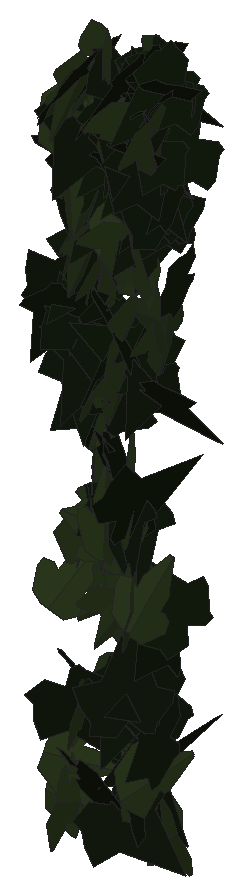
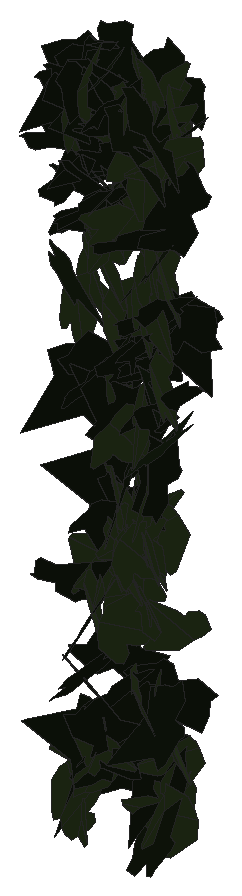
# SketchUp Ruby script. Lengths in inches.
U = 1.inch
M = Sketchup.active_model
def pt(a) = Geom::Point3d.new(a.map { |v| v * U })
def face(e, loops, mat)
  f = e.add_face(loops[0].map { |a| pt(a) })
  loops[1..].each { |l| e.add_face(l.map { |a| pt(a) }).erase! }
  f.material = f.back_material = mat if mat
  f
end
# faces: each face lists its corners as indices into pts; further lists are holes
def faces(e, pts, list, mat = nil) = list.each { |f| face(e, (f[0].is_a?(Array) ? f : [f]).map { |l| l.map { |i| pts[i] } }, mat) }
# xy, xz, yz: faces in a plane at the given z, y or x. An outline is a flat list of corners, or four numbers for a rectangle; further outlines are holes
def ring(l) = l.size == 4 ? [[l[0], l[1]], [l[2], l[1]], [l[2], l[3]], [l[0], l[3]]] : l.each_slice(2).to_a
def flat(e, list, mat, &to3) = list.each { |f| face(e, (f[0].is_a?(Array) ? f : [f]).map { |l| ring(l).map { |u, v| to3.(u, v) } }, mat) }
def xy(e, z, list, mat = nil) = flat(e, list, mat) { |x, y| [x, y, z] }
def xz(e, y, list, mat = nil) = flat(e, list, mat) { |x, z| [x, y, z] }
def yz(e, x, list, mat = nil) = flat(e, list, mat) { |y, z| [x, y, z] }
def lines(e, pts, list) = list.each { |a, b| e.add_line(pt(pts[a]), pt(pts[b])) }
# prism: a flat outline (further loops are holes) pulled along v
def prism(e, loops, v, mat = nil)
  f = face(e, loops, mat); d = Geom::Vector3d.new(v.map { |x| x * U })
  f.pushpull(f.normal.samedirection?(d) ? d.length : -d.length)
end
def box(e, o, s, mat = nil) = prism(e, [[o, [o[0] + s[0], o[1], o[2]], [o[0] + s[0], o[1] + s[1], o[2]], [o[0], o[1] + s[1], o[2]]]], [0, 0, s[2]], mat)
def at(x, y, z, deg = 0) = Geom::Transformation.translation(pt([x, y, z])) * Geom::Transformation.rotation(ORIGIN, Z_AXIS, deg.degrees)
def axes(o, x, y, z) = Geom::Transformation.new([*x, 0, *y, 0, *z, 0, *pt(o).to_a, 1])
def part(name) = M.definitions.add(name)
# library, detail: a bought-in or finely detailed component or shape, given as its bounding box
def library(name, o, s) = part(name).tap { |d| box(d.entities, o, s) }
def detail(e, o, s) = box(e.add_group.entities, o, s)
def put(e, d, t, mat = nil) = e.add_instance(d, t).tap { |i| i.material = mat if mat }
def group(e, t, mat = nil) = e.add_group.tap { |g| g.transformation = t; g.material = mat if mat }.entities
root = M.entities
M.materials.add("efeu1").color = [18, 25, 13]
M.materials.add("efeu2").color = [43, 57, 29]
c1 = part("ivyleaf_10")
p = [[0,0.5,-0.03],[-0.0625,2.02,-0.43],[-0.19,2.01,-0.46],[-0.54,1.05,-0.29],[-0.52,0.625,-0.18],[-0.83,0.76,-0.28],
  [-1.16,0.64,-0.33],[-1.15,0.33,-0.24],[-0.77,-0.39,0.02],[-0.3,-0.51,0.16],[0.04,-0.48,0.23],[-0.02,2.01,-0.4375],
  [-0.06,2.01,-0.43],[0.04,-0.49,0.23],[0.67,-0.49,0.14],[1.38,0.36,-0.2],[1.375,0.51,-0.24],[0.81,0.65,-0.19],
  [0.62,0.59,-0.15],[0.6,1.09,-0.28],[0.5,1.23,-0.31]]
faces(c1.entities,p,[[0,1,2,3,4,5,6,7,8,9,10],[11,12,0,13,14,15,16,17,18,19,20]],"efeu2")
c2 = part("ivyleaf_9")
p = [[1.54,2.16,1.25],[1.36,2.04,1.19],[-0.21,0.99,0.68],[-0.71,1.11,0.82],[-0.85,0.86,0.67],[-0.8,0.17,0.21],
  [-0.9,-0.01,0.1],[-0.67,-0.16,-0.02],[-0.08,-0.08,-0.05],[-0.03,-0.6,-0.4],[0.65,-0.88,-0.66],[0.83,-0.6,-0.49],
  [1.29,-0.42,-0.43],[1.8125,-0.07,-0.26],[1.21,0.44,0.15]]
faces(c2.entities,p,[[0,1,2,3,4,5,6,7,8,9,10,11,12,13,14]],"efeu1")
put(root,c1,axes([534.45,133.85,189.87],[0.52403,0.27008,-0.47127],[0.36222,0.31422,0.58285],[0.40477,-0.63085,0.08854]))
put(root,c1,axes([534.74,134.3125,200.51],[0.41186,-0.70817,0.08456],[0.03957,-0.07481,-0.81922],[0.71211,0.41374,-0.00339]))
put(root,c1,axes([534.41,133.79,203.66],[0.12614,-0.20221,-0.804],[0.55612,0.62378,-0.06963],[0.61485,-0.52272,0.22793]))
put(root,c2,axes([535.04,133.58,198.78],[0.17028,0.49004,-0.61455],[-0.1647,-0.5926,-0.51818],[-0.76856,0.23557,-0.02512]))
put(root,c2,axes([534.1,134.25,202.35],[0.60101,0.32484,-0.52857],[0.4439,0.28896,0.68233],[0.43342,-0.74639,0.03411]))
put(root,c1,axes([535.39,134.32,199.52],[-0.544,0.12691,0.70025],[-0.69799,0.07673,-0.55616],[-0.13878,-0.8834,0.05229]))
put(root,c2,axes([534.48,134.38,201.37],[0.55114,-0.55181,-0.28459],[-0.13721,0.26288,-0.77544],[0.60552,0.56182,0.08331]))
put(root,c2,axes([534.75,134.99,195.28],[-0.3652,-0.47282,0.58309],[0.04509,-0.66108,-0.50781],[0.74935,-0.19065,0.31474]))
put(root,c2,axes([534.9375,135.01,199.4],[-0.46878,-0.60321,0.25493],[-0.08946,-0.25158,-0.7598],[0.64872,-0.47058,0.07943]))
put(root,c2,axes([534.58,133.8,198.375],[-0.49104,0.09387,0.70212],[0.64899,-0.28279,0.49169],[0.28391,0.80878,0.09043]))
put(root,c1,axes([534.78,134.17,204.3125],[0.05286,-0.68254,0.49372],[0.22578,-0.46511,-0.66717],[0.81157,0.17385,0.15345]))
put(root,c2,axes([534.39,134.46,187.62],[0.7773,-0.31884,0.07692],[0.0716,-0.02813,-0.84015],[0.32007,0.78059,0.00114]))
put(root,c2,axes([535.29,134.4,205.12],[-0.42132,0.70206,0.02308],[-0.00734,0.02251,-0.81876],[-0.7024,-0.42135,-0.00528]))
put(root,c1,axes([534.97,133.59,205.01],[0.30351,-0.80065,-0.01801],[-0.00368,0.01787,-0.85624],[0.80084,0.30352,0.00289]))
put(root,c1,axes([534.88,134.4,197.35],[0.39562,-0.71526,0.2599],[0.12085,-0.23016,-0.81736],[0.75135,0.41363,-0.00538]))
put(root,c2,axes([534.78,134.59,196.69],[-0.09569,-0.80257,-0.06848],[0.00675,0.06816,-0.80825],[0.80546,-0.09592,-0.00137]))
put(root,c2,axes([535.03,134.625,183.49],[0.5026,-0.66038,0.08772],[-0.05245,0.07031,0.82988],[-0.66411,-0.50533,0.00084]))
put(root,c1,axes([534.73,133.62,185.76],[0.53384,-0.47088,-0.34601],[0.29212,-0.19085,0.71041],[-0.50609,-0.60687,0.04506]))
put(root,c1,axes([535.21,134.05,201.01],[0.1399,-0.80695,-0.17252],[-0.03873,0.16837,-0.81893],[0.82428,0.14487,-0.00919]))
put(root,c2,axes([534.51,134.6,194.55],[0.57855,-0.08826,-0.5894],[0.593,0.00323,0.58159],[-0.05951,-0.8259,0.06526]))
put(root,c1,axes([535.06,133.93,205.06],[0.13574,-0.56849,0.65049],[0.25305,-0.60342,-0.58016],[0.826,0.27828,0.07083]))
put(root,c2,axes([535.36,132.76,205.13],[0.09715,0.69874,0.51085],[0.06789,0.50632,-0.70545],[-0.8629,0.1185,0.00201]))
put(root,c1,axes([535.33,134.4,203.61],[-0.61646,-0.53676,-0.00082],[0.00113,-0.00005,-0.81739],[0.53676,-0.61646,0.00078]))
put(root,c1,axes([535.13,134.43,192.49],[0.43438,-0.61985,0.27564],[0.1487,-0.23234,-0.75682],[0.66187,0.459,-0.01087]))
put(root,c1,axes([535.3,135,192.54],[-0.11993,-0.561,0.57544],[0.05662,-0.58626,-0.55975],[0.80165,-0.04252,0.12562]))
put(root,c1,axes([535.32,134.2,200.41],[0.06181,-0.75177,0.34655],[0.05702,-0.34282,-0.75385],[0.82584,0.07993,0.02611]))
put(root,c2,axes([535.12,134.12,203.55],[-0.2093,-0.74721,0.42147],[0.03089,-0.44011,-0.76492],[0.85732,-0.16656,0.13045]))
put(root,c1,axes([535.35,132.92,184.7],[0.00533,-0.44816,-0.88066],[0.09786,0.87658,-0.4455],[0.98328,-0.08481,0.04911]))
put(root,c1,axes([535.19,133.44,202.61],[-0.12517,0.77309,-0.29128],[0.07052,-0.28353,-0.78283],[-0.82313,-0.14186,-0.02277]))
put(root,c1,axes([535.83,134.16,192.75],[0.27188,-0.2591,-0.81608],[-0.58497,0.56904,-0.37556],[0.62524,0.64506,0.0035]))
put(root,c2,axes([535.05,134.04,198.3125],[0.05115,-0.79256,-0.34222],[0.05639,0.34515,-0.79093],[0.86144,0.02446,0.07209]))
put(root,c1,axes([535.45,134.23,196.38],[0.14509,-0.66521,-0.44848],[-0.00339,0.45525,-0.67634],[0.80227,0.12223,0.07825]))
put(root,c1,axes([535.44,134.34,199.56],[0.19712,-0.7967,-0.07406],[0.00193,0.07674,-0.82048],[0.80014,0.19609,0.02022]))
put(root,c1,axes([534.78,133.63,184.35],[-0.09326,0.00454,-0.8347],[0.82927,-0.09524,-0.09318],[-0.09515,-0.83448,0.00609]))
put(root,c2,axes([535.81,134.47,204.6],[-0.44527,0.69545,-0.09822],[0.04461,-0.08806,-0.82572],[-0.70093,-0.44739,0.00984]))
put(root,c1,axes([534.93,134.68,190.49],[0.41487,-0.34005,-0.64694],[0.53884,-0.36029,0.53491],[-0.49379,-0.67885,0.04017]))
put(root,c1,axes([535.29,134.41,193.85],[-0.21124,0.57267,-0.58428],[0.12656,-0.57331,-0.60767],[-0.80828,-0.23943,0.05755]))
put(root,c2,axes([535.5625,135.1,201.4],[-0.55139,-0.59264,0.17754],[0.02495,-0.25893,-0.78683],[0.61816,-0.51817,0.19012]))
put(root,c1,axes([535.48,134.28,205.96],[0.72123,-0.45576,-0.02408],[0.01647,0.07099,-0.85039],[0.4561,0.71813,0.06878]))
put(root,c1,axes([535.1,133.1,185.85],[-0.12333,-0.24858,-0.70562],[0.66826,0.2849,-0.21717],[0.33633,-0.65722,0.17275]))
put(root,c1,axes([535.75,135.1,190.17],[-0.05903,-0.28963,0.71903],[-0.11167,-0.71041,-0.29532],[0.76708,-0.1257,0.01234]))
put(root,c2,axes([536.01,134.62,197.25],[-0.35064,0.06385,0.72928],[-0.60611,-0.47881,-0.2495],[0.41056,-0.65234,0.25451]))
put(root,c2,axes([535.58,134.05,197.5],[-0.31814,-0.73627,0.1545],[-0.07534,-0.13572,-0.80192],[0.74852,-0.32659,-0.01505]))
put(root,c1,axes([535.66,134.83,192.23],[0.21787,-0.73463,0.17048],[0.02623,-0.16996,-0.76593],[0.7537,0.21827,-0.02263]))
put(root,c2,axes([536.1,133.27,196.9],[-0.20759,0.6106,0.49817],[-0.16073,0.47153,-0.64492],[-0.77148,-0.26254,0.00031]))
put(root,c2,axes([535.73,134.3,194.77],[0.49749,-0.25214,-0.63948],[-0.57027,0.28935,-0.55773],[0.38379,0.75677,0.00019]))
put(root,c1,axes([535.84,134.87,195.74],[0.2349,0.59012,-0.50006],[-0.30123,-0.41156,-0.62718],[-0.71243,0.36859,0.1003]))
put(root,c1,axes([535.84,132.96,187.53],[0.12181,-0.46759,-0.59193],[-0.04194,0.59447,-0.47823],[0.75317,0.10873,0.0691]))
put(root,c2,axes([535.35,133.12,187.79],[-0.16405,-0.2719,-0.80747],[0.39272,0.70562,-0.31739],[0.75612,-0.42548,-0.01035]))
put(root,c1,axes([535.54,134.37,187.91],[0.55141,-0.44206,0.40539],[0.29662,-0.27763,-0.70622],[0.52131,0.62555,-0.02696]))
put(root,c2,axes([535.78,133.05,185.69],[0.80337,0.10893,-0.41678],[-0.41288,-0.05692,-0.81072],[-0.12291,0.90325,-0.00082]))
put(root,c1,axes([536.17,133.91,192.22],[0.08272,0.50797,0.62453],[-0.1831,-0.5995,0.51186],[0.78394,-0.19362,0.05365]))
put(root,c2,axes([536.2,134.93,203.62],[-0.71044,-0.41412,0.06534],[-0.04648,-0.04997,-0.82209],[0.41666,-0.71169,0.0197]))
put(root,c1,axes([535.54,133.47,192.48],[-0.46813,-0.20873,-0.75076],[0.69684,0.27985,-0.51231],[0.34875,-0.83933,0.01589]))
put(root,c2,axes([535.67,135.08,202.9375],[0.05804,-0.7547,0.31294],[0.0954,-0.30532,-0.75402],[0.81142,0.08988,0.06626]))
put(root,c2,axes([536.74,134.52,186.15],[-0.23345,0.03377,0.87946],[-0.85951,0.18695,-0.23533],[-0.18929,-0.8905,-0.01605]))
put(root,c2,axes([535.75,134.16,195.55],[-0.24262,-0.03034,0.81647],[0.8167,0.01516,0.24325],[-0.02318,0.85162,0.02476]))
put(root,c1,axes([535.94,134.57,205.01],[-0.51552,0.48018,-0.43412],[0.28962,-0.32524,-0.70366],[-0.57893,-0.59029,0.03456]))
put(root,c2,axes([535.88,134.76,205.23],[0.09666,-0.82403,-0.08937],[-0.00091,0.08987,-0.82962],[0.82886,0.09619,0.00952]))
put(root,c1,axes([536.29,134.29,193.21],[0.60617,-0.46995,0.37037],[-0.29828,0.21971,0.76696],[-0.51871,-0.67554,-0.00821]))
put(root,c1,axes([536.43,134,193.19],[0.61178,-0.44278,-0.34263],[-0.25419,0.23253,-0.75435],[0.49884,0.66152,0.03583]))
put(root,c1,axes([535.72,134.29,191.68],[0.44334,-0.22823,-0.69233],[0.63759,-0.27142,0.49776],[-0.35339,-0.77602,0.02952]))
put(root,c1,axes([536.48,133.05,192.5],[-0.06222,0.74109,-0.54363],[-0.09608,0.53665,0.74256],[0.91407,0.10685,0.04105]))
put(root,c2,axes([536.8,134.68,197.01],[-0.11574,0.10753,0.7993],[-0.77574,-0.23573,-0.08062],[0.22062,-0.77247,0.13587]))
put(root,c1,axes([536.42,133.99,197],[0.05315,-0.81817,0.0626],[-0.00221,-0.06288,-0.81987],[0.82056,0.05283,-0.00626]))
put(root,c2,axes([535.78,134.1,187],[0.60485,-0.42426,0.40784],[0.33601,-0.23118,-0.7388],[0.48315,0.69191,0.00323]))
put(root,c1,axes([536.12,134.13,201.32],[0.34488,0.63738,0.44975],[0.23058,0.38648,-0.72452],[-0.74522,0.41455,-0.01604]))
put(root,c2,axes([535.96,134.23,198.17],[0.18049,-0.54099,0.65103],[0.28486,-0.58802,-0.5676],[0.7971,0.33264,0.05543]))
put(root,c1,axes([536.31,134.09,204.65],[0.87252,0.0776,0.13545],[0.13491,0.01208,-0.87597],[-0.07854,0.88289,0.00008]))
put(root,c1,axes([536.63,133.55,190.65],[-0.74274,-0.32233,-0.02965],[0.02718,0.01184,-0.80967],[0.32255,-0.74324,-0.00004]))
put(root,c1,axes([537.11,134.52,186.21],[-0.20003,0.06176,0.72495],[-0.69683,-0.23253,-0.17246],[0.20929,-0.71519,0.11868]))
put(root,c2,axes([536.47,134.37,187.66],[-0.26203,-0.74455,0.21268],[-0.02041,-0.21781,-0.78765],[0.77406,-0.25778,0.05123]))
put(root,c1,axes([536.46,134.14,190.34],[-0.03143,-0.25352,0.78401],[0.28058,-0.74099,-0.22835],[0.77474,0.25807,0.11451]))
put(root,c2,axes([536.35,133.88,193.33],[-0.42638,-0.30085,-0.56503],[0.44159,0.35327,-0.52133],[0.46344,-0.61341,-0.02311]))
put(root,c2,axes([536.61,134.75,204.14],[-0.47367,-0.67247,0.08596],[-0.02857,-0.08497,-0.82215],[0.67734,-0.47385,0.02543]))
put(root,c1,axes([536.88,134.6,204.38],[-0.43958,-0.46717,0.51575],[-0.2221,-0.48394,-0.62765],[0.65948,-0.47437,0.13239]))
put(root,c1,axes([536.53,134.16,198.58],[0.26539,-0.66728,0.49053],[0.17937,-0.45656,-0.71811],[0.80852,0.32031,-0.0017]))
put(root,c2,axes([536.39,134.23,193.13],[-0.06759,-0.86837,-0.28247],[0.03173,0.28084,-0.87094],[0.9126,-0.07408,0.00937]))
put(root,c1,axes([536.82,133.61,204.7],[-0.26789,-0.79434,0.18451],[-0.03942,-0.18137,-0.83805],[0.81453,-0.27003,0.02013]))
put(root,c2,axes([536.375,134.06,204.08],[-0.08061,-0.77865,0.31745],[0.14974,-0.3271,-0.7643],[0.82744,-0.01667,0.16924]))
put(root,c1,axes([536.9,133.43,201.37],[-0.57458,-0.57608,0.05605],[-0.04391,-0.03537,-0.81361],[0.57713,-0.57622,-0.0061]))
put(root,c2,axes([536.96,133.99,205.94],[-0.42946,0.26931,-0.65713],[0.29668,-0.62969,-0.45195],[-0.64524,-0.46877,0.22957]))
put(root,c1,axes([537.07,134.125,200.4],[0.62646,-0.38982,-0.50707],[-0.4186,0.28677,-0.73761],[0.48359,0.75322,0.0184]))
put(root,c2,axes([536.99,134.77,205.85],[-0.24369,0.43028,-0.67795],[0.30939,-0.60347,-0.49422],[-0.74097,-0.39349,0.0166]))
put(root,c2,axes([536.74,134.95,196.86],[-0.1633,-0.71639,0.31664],[-0.04474,-0.31439,-0.73437],[0.78197,-0.16759,0.02411]))
put(root,c1,axes([536.75,134.79,190.625],[0.42161,-0.56845,0.36887],[0.25414,-0.27008,-0.7067],[0.62818,0.49079,0.03834]))
put(root,c1,axes([536.63,135.15,205.4375],[-0.04043,-0.18623,0.80476],[0.49553,-0.65011,-0.12555],[0.66088,0.47606,0.14337]))
put(root,c1,axes([537.13,134.17,184.85],[-0.00403,0.83102,0.18644],[-0.03621,-0.18644,0.83024],[0.85091,-0.004,0.03622]))
put(root,c2,axes([537.1,133.59,203.9],[-0.26303,0.65465,-0.57528],[-0.31638,0.48818,0.7002],[0.81204,0.40225,0.08646]))
put(root,c2,axes([537.05,134.8,201.625],[-0.39352,-0.6603,0.30634],[-0.08867,-0.30217,-0.7652],[0.72248,-0.39674,0.07295]))
put(root,c2,axes([536.62,133.48,203.48],[0.81078,0.19878,0.19434],[0.18245,0.0716,-0.8344],[-0.20975,0.83067,0.02541]))
put(root,c2,axes([537.26,133.1875,187.66],[-0.77322,-0.1518,0.34435],[0.34822,0.00976,0.78621],[-0.1427,0.84637,0.0527]))
put(root,c2,axes([537.37,134.78,205.55],[-0.7775,-0.33646,-0.01402],[0.01307,0.0051,-0.84718],[0.3365,-0.77761,0.00051]))
put(root,c1,axes([537.125,134.9,204.57],[0.07099,-0.78043,0.27256],[0.11558,-0.2615,-0.77888],[0.81854,0.1046,0.08634]))
put(root,c2,axes([537.09,134.77,201.67],[-0.28391,-0.75887,0.05999],[-0.03812,-0.04977,-0.81003],[0.76028,-0.28588,-0.01822]))
put(root,c1,axes([537.23,133.46,190.97],[0.10657,-0.01039,-0.84988],[0.03756,0.85575,-0.00575],[0.84911,-0.03655,0.10692]))
put(root,c1,axes([537.38,133.17,190.84],[0.06122,-0.33489,-0.79122],[-0.13667,0.77933,-0.34043],[0.84823,0.14974,0.00225]))
put(root,c2,axes([536.89,133.3,193.22],[0.08116,0.08448,0.90621],[0.68451,0.59395,-0.11667],[-0.59984,0.68923,-0.01053]))
put(root,c2,axes([536.84,134.85,205.16],[0.04466,-0.73931,0.38794],[0.14317,-0.37596,-0.73296],[0.82254,0.10558,0.10651]))
put(root,c2,axes([536.99,134.92,189.46],[-0.05012,-0.58493,0.65199],[-0.01253,-0.65251,-0.58636],[0.87583,-0.04281,0.02892]))
put(root,c2,axes([537.46,133.96,204.92],[0.04866,0.83979,-0.05518],[-0.00375,-0.05506,-0.8412],[-0.8416,0.04881,0.00056]))
put(root,c2,axes([537.7,134.47,202.32],[-0.81294,0.05759,0.06096],[-0.06063,0.00688,-0.81497],[-0.05794,-0.81519,-0.00257]))
put(root,c1,axes([537.47,133.52,200.23],[-0.54615,0.66778,-0.05249],[-0.04055,0.03465,0.86262],[0.66861,0.54757,0.00943]))
put(root,c2,axes([537.51,134.14,203.86],[-0.61129,-0.542,0.13138],[-0.09877,-0.08663,-0.81696],[0.54888,-0.61921,-0.00069]))
put(root,c2,axes([536.88,133.06,184.95],[0.13655,-0.44334,-0.72006],[0.2742,0.71319,-0.38711],[0.7999,-0.16879,0.25562]))
put(root,c1,axes([537.9375,133.52,199.23],[-0.24739,0.17221,0.81277],[-0.77578,0.25564,-0.29029],[-0.29736,-0.81021,0.08116]))
put(root,c2,axes([537.51,134.7,187.7],[-0.41575,-0.29304,0.63154],[-0.24194,-0.62892,-0.4511],[0.65283,-0.4197,0.23502]))
put(root,c2,axes([537.33,133.81,185.29],[0.28876,-0.37027,-0.64372],[-0.37468,0.52368,-0.4693],[0.64116,0.47278,0.01567]))
put(root,c2,axes([537.27,133.8125,185.74],[-0.05425,0.76908,-0.33056],[-0.02458,0.32965,0.77099],[0.83675,0.05955,0.00122]))
put(root,c1,axes([537.47,134.59,183.83],[-0.13046,0.33759,0.69621],[0.18858,-0.67087,0.36064],[0.75041,0.22728,0.0304]))
put(root,c2,axes([537.18,133.53,203.53],[0.32497,-0.6411,-0.46545],[-0.0609,0.48138,-0.70556],[0.7899,0.30086,0.13709]))
put(root,c2,axes([537.82,134.75,199.85],[-0.67961,0.3304,-0.2947],[0.23995,-0.17886,-0.75387],[-0.37208,-0.71884,0.05212]))
put(root,c2,axes([537.23,134.02,205.24],[0.72201,0.33888,0.21192],[0.16873,0.13824,-0.79591],[-0.36233,0.73967,0.05166]))
put(root,c2,axes([537.78,134.64,205.49],[-0.5239,-0.5633,0.36182],[-0.24952,-0.26204,-0.76926],[0.62126,-0.58027,-0.00385]))
put(root,c2,axes([537.17,134.17,196.51],[0.79814,0.12183,0.11698],[0.11241,0.03855,-0.80712],[-0.12606,0.80575,0.02093]))
put(root,c1,axes([537.66,134.15,198.7],[-0.00973,-0.82209,-0.07048],[0.01067,0.07035,-0.82209],[0.82503,-0.01061,0.0098]))
put(root,c1,axes([537.41,133.18,185.59],[0.11425,0.11293,-0.94264],[0.40152,0.8546,0.15105],[0.86029,-0.41386,0.05469]))
put(root,c2,axes([537.94,134.01,202.82],[-0.77034,0.19179,-0.20522],[0.18643,-0.09896,-0.79232],[-0.21009,-0.79104,0.04936]))
put(root,c2,axes([538.21,134.26,190.23],[-0.69753,-0.34063,-0.20475],[-0.1844,-0.089,0.77626],[-0.35207,0.7215,-0.00091]))
put(root,c2,axes([537.91,135.04,203.67],[-0.66886,-0.45882,0.18135],[-0.0939,-0.18154,-0.80561],[0.48434,-0.66881,0.09426]))
put(root,c1,axes([537.59,133.08,190.68],[0.2605,0.49924,-0.67993],[0.21646,0.64822,0.55889],[0.81529,-0.33162,0.06887]))
put(root,c2,axes([537.9,133.88,201.7],[-0.44006,-0.49381,0.58323],[0.38507,0.43805,0.66143],[-0.66009,0.58474,-0.00296]))
put(root,c1,axes([538.29,133.8,184.29],[-0.52103,0.13899,0.70175],[-0.67456,0.19362,-0.53919],[-0.23821,-0.85231,-0.00805]))
put(root,c2,axes([538.27,133.46,187.28],[-0.83801,0.35325,0.03998],[-0.03712,0.01487,-0.90942],[-0.35357,-0.83883,0.00071]))
put(root,c1,axes([537.85,133.27,204.73],[0.00417,-0.81409,-0.25696],[0.06069,0.2566,-0.81195],[0.85153,-0.0143,0.05912]))
